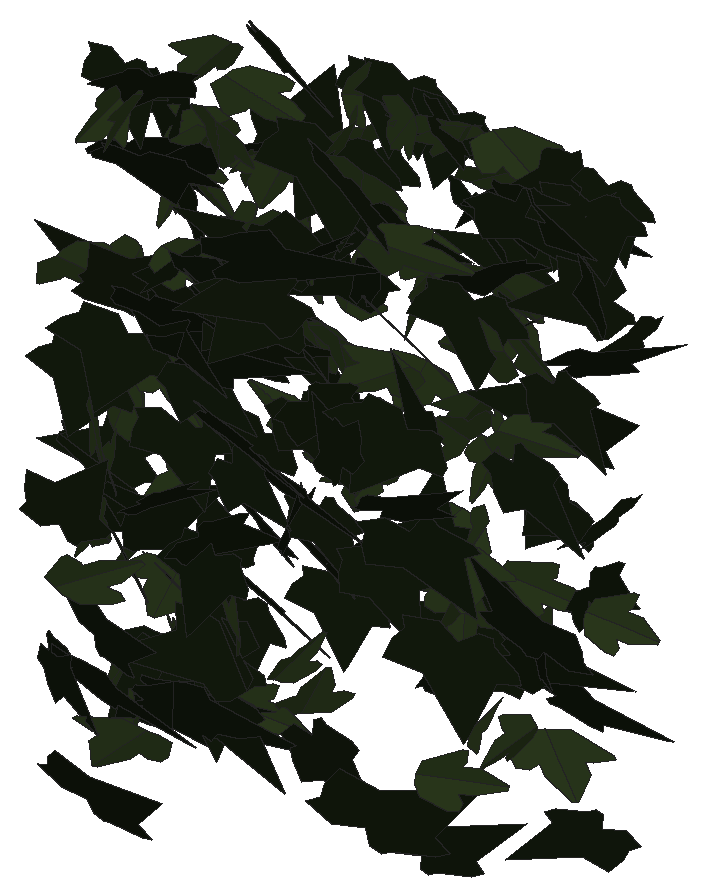
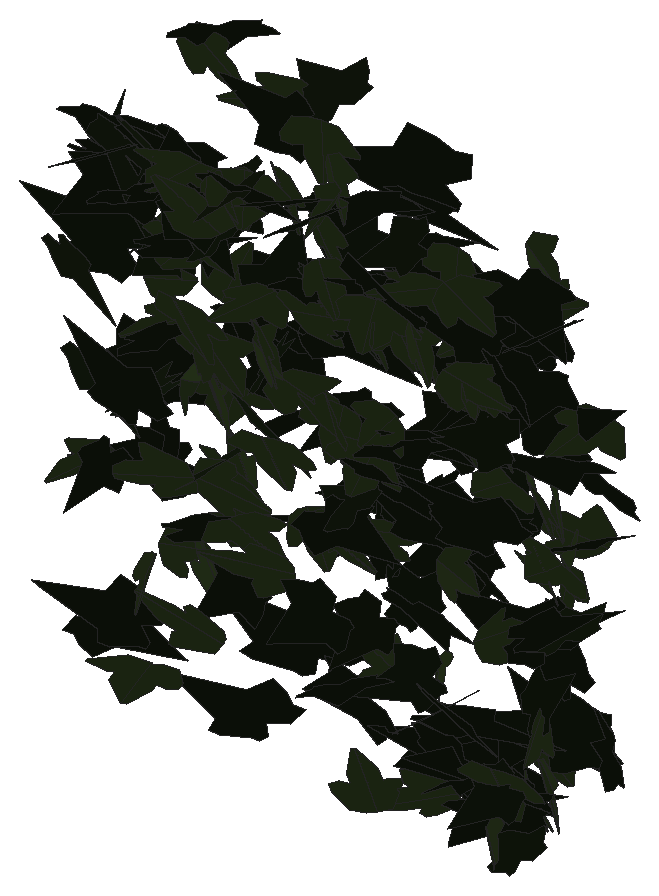
# SketchUp Ruby script. Lengths in millimetres.
U = 1.mm
M = Sketchup.active_model
def pt(a) = Geom::Point3d.new(a.map { |v| v * U })
def face(e, loops, mat)
  f = e.add_face(loops[0].map { |a| pt(a) })
  loops[1..].each { |l| e.add_face(l.map { |a| pt(a) }).erase! }
  f.material = f.back_material = mat if mat
  f
end
# faces: each face lists its corners as indices into pts; further lists are holes
def faces(e, pts, list, mat = nil) = list.each { |f| face(e, (f[0].is_a?(Array) ? f : [f]).map { |l| l.map { |i| pts[i] } }, mat) }
# xy, xz, yz: faces in a plane at the given z, y or x. An outline is a flat list of corners, or four numbers for a rectangle; further outlines are holes
def ring(l) = l.size == 4 ? [[l[0], l[1]], [l[2], l[1]], [l[2], l[3]], [l[0], l[3]]] : l.each_slice(2).to_a
def flat(e, list, mat, &to3) = list.each { |f| face(e, (f[0].is_a?(Array) ? f : [f]).map { |l| ring(l).map { |u, v| to3.(u, v) } }, mat) }
def xy(e, z, list, mat = nil) = flat(e, list, mat) { |x, y| [x, y, z] }
def xz(e, y, list, mat = nil) = flat(e, list, mat) { |x, z| [x, y, z] }
def yz(e, x, list, mat = nil) = flat(e, list, mat) { |y, z| [x, y, z] }
def lines(e, pts, list) = list.each { |a, b| e.add_line(pt(pts[a]), pt(pts[b])) }
# prism: a flat outline (further loops are holes) pulled along v
def prism(e, loops, v, mat = nil)
  f = face(e, loops, mat); d = Geom::Vector3d.new(v.map { |x| x * U })
  f.pushpull(f.normal.samedirection?(d) ? d.length : -d.length)
end
def box(e, o, s, mat = nil) = prism(e, [[o, [o[0] + s[0], o[1], o[2]], [o[0] + s[0], o[1] + s[1], o[2]], [o[0], o[1] + s[1], o[2]]]], [0, 0, s[2]], mat)
def at(x, y, z, deg = 0) = Geom::Transformation.translation(pt([x, y, z])) * Geom::Transformation.rotation(ORIGIN, Z_AXIS, deg.degrees)
def axes(o, x, y, z) = Geom::Transformation.new([*x, 0, *y, 0, *z, 0, *pt(o).to_a, 1])
def part(name) = M.definitions.add(name)
# library, detail: a bought-in or finely detailed component or shape, given as its bounding box
def library(name, o, s) = part(name).tap { |d| box(d.entities, o, s) }
def detail(e, o, s) = box(e.add_group.entities, o, s)
def put(e, d, t, mat = nil) = e.add_instance(d, t).tap { |i| i.material = mat if mat }
def group(e, t, mat = nil) = e.add_group.tap { |g| g.transformation = t; g.material = mat if mat }.entities
root = M.entities
M.materials.add("efeu1").color = [18, 25, 13]
M.materials.add("efeu2").color = [43, 57, 29]
c1 = part("ivyleaf_9")
p = [[39.1,54.8,31.7],[34.5,51.8,30.2],[-5.3,25.2,17.3],[-17.9,28.3,20.9],[-21.6,21.7,17],[-20.2,4.3,5.3],
  [-22.9,-0.3,2.5],[-17.1,-4,-0.6],[-2,-2.1,-1.2],[-0.7,-15.4,-10.1],[16.6,-22.3,-16.7],[21.1,-15.1,-12.5],
  [32.7,-10.7,-11],[46.1,-1.8,-6.6],[30.8,11.2,3.8]]
faces(c1.entities,p,[[0,1,2,3,4,5,6,7,8,9,10,11,12,13,14]],"efeu1")
c2 = part("ivyleaf_10")
p = [[0,12.8,-0.8],[-1.5,51.3,-10.9],[-4.9,51,-11.6],[-13.6,26.5,-7.3],[-13.2,15.9,-4.6],[-21.1,19.3,-7.2],
  [-29.5,16.3,-8.3],[-29.2,8.3,-6.2],[-19.7,-9.8,0.5],[-7.6,-13,4],[1,-12.2,5.8],[-0.4,51.1,-11.1],
  [-1.5,51.1,-10.9],[1,-12.4,5.9],[16.9,-12.4,3.5],[35.1,9.1,-5.1],[35,12.9,-6.1],[20.5,16.4,-4.9],
  [15.8,15,-3.8],[15.3,27.6,-7.1],[12.8,31.3,-7.8]]
faces(c2.entities,p,[[0,1,2,3,4,5,6,7,8,9,10],[11,12,0,13,14,15,16,17,18,19,20]],"efeu2")
put(root,c1,axes([5512.2,727.9,3383.8],[-0.13252,-1.17881,0.07972],[-0.00116,-0.07982,-1.18086],[2.24864,-0.06951,0.00409]))
put(root,c2,axes([5531.2,716.1,3146.5],[1.27078,-0.95438,0.07013],[0.07944,-0.05639,-1.16476],[1.81955,0.66901,0.00188]))
put(root,c1,axes([5537.2,633.9,3034.5],[-1.01754,-1.05883,0.3155],[-0.00054,-0.35036,-1.17632],[2.10271,-0.51247,0.15237]))
put(root,c1,axes([5526.2,783.4,3340.5],[-0.99944,0.03385,-1.03029],[1.91291,-0.23997,-0.52018],[-0.4357,-1.13123,0.07952]))
put(root,c1,axes([5572,679.8,2911.2],[-0.74,-0.15956,1.27167],[-1.90352,-0.7932,-0.40533],[1.52527,-1.06732,0.11112]))
put(root,c1,axes([5542.4,700.6,3305.1],[1.32687,0.89042,-0.05971],[-0.03543,-0.06124,-1.13065],[-1.69808,0.69704,-0.02307]))
put(root,c2,axes([5531.4,597.9,3193.9],[-1.11357,-0.5992,-0.91061],[1.1456,0.68404,-0.83688],[1.72964,-0.83884,-0.03197]))
put(root,c2,axes([5553.4,657.8,3375.6],[0.26095,0.41133,-1.16672],[-0.63142,-1.11863,-0.43336],[-2.2682,0.35873,-0.01359]))
put(root,c2,axes([5554.2,678.3,2790.1],[-0.03114,-0.60966,-1.0137],[0.17755,1.00997,-0.60892],[2.24429,-0.08836,0.03411]))
put(root,c2,axes([5529.6,675.3,3023.9],[1.76327,-0.17198,0.81089],[1.5071,-0.1759,-0.94206],[0.4664,1.21859,-0.02154]))
put(root,c1,axes([5538.6,648.5,2908.2],[-0.17529,-1.05107,0.83425],[0.48012,-0.83486,-1.02399],[2.50838,0.08635,0.2543]))
put(root,c1,axes([5582.3,685,3412.5],[0.33493,0.97332,-0.77439],[-0.2593,-0.76231,-0.9891],[-2.35296,0.22255,-0.00123]))
put(root,c2,axes([5571.2,748.2,3240.6],[1.16552,-0.96879,0.09099],[0.07584,-0.08245,-1.14607],[1.85036,0.61361,-0.01034]))
put(root,c1,axes([5535.4,780.1,3243.5],[1.4862,-0.6817,0.42925],[0.59094,-0.29694,-1.03643],[1.41474,0.84017,-0.01802]))
put(root,c2,axes([5578,734,2732.6],[2.16816,-0.12358,-0.14672],[-0.27506,0.02812,-1.14583],[0.24007,1.14828,0.01227]))
put(root,c1,axes([5596.4,641.2,2778.9],[0.18517,-0.91045,0.92088],[-0.09628,0.9201,0.91503],[-2.4627,-0.10443,0.03347]))
put(root,c2,axes([5599.5,785,3314.6],[-0.70687,-0.62185,0.894],[-0.69244,-0.81944,-0.72113],[1.9535,-0.51547,0.06788]))
put(root,c2,axes([5570.4,649.4,2973.9],[1.62253,-0.79065,0.01438],[-0.0173,0.01134,1.16272],[-1.50491,-0.85257,0.00213]))
put(root,c1,axes([5618.6,627.4,3164.2],[0.43411,-0.02764,1.34009],[-2.50693,0.24697,0.2293],[-0.47214,-1.33674,0.01465]))
put(root,c2,axes([5595.1,724.3,2642.3],[0.17713,-0.01007,-1.11887],[-0.50576,1.09041,-0.03192],[2.06859,0.26746,0.088]))
put(root,c1,axes([5560.1,739.4,2726.4],[1.93704,-0.46994,-0.30845],[-0.53555,0.12637,-1.12103],[0.92614,1.05596,-0.00311]))
put(root,c2,axes([5558.1,611.9,2984.7],[0.23797,-0.45101,1.17667],[1.55541,-0.87103,-0.4207],[1.82554,0.80093,0.20506]))
put(root,c1,axes([5550.1,546.1,2698.4],[0.16552,-0.22108,-1.27596],[2.39043,-0.29695,0.13706],[-0.60004,-1.24397,0.19405]))
put(root,c2,axes([5596.6,615.6,2678],[0.71983,-1.08268,-0.50877],[-0.2415,0.49427,-1.14616],[2.26389,0.39698,0.0395]))
put(root,c2,axes([5592.5,764.3,3299.9],[-0.00034,-0.92288,0.72446],[0.31149,-0.71739,-0.91384],[2.21112,0.10092,0.12885]))
put(root,c1,axes([5568.4,701.6,2609],[0.13885,-0.79141,0.86504],[0.44291,-0.8397,-0.78785],[2.187,0.2203,0.10463]))
put(root,c2,axes([5614.9,770.9,3424.3],[-0.64439,-0.9713,0.66241],[-0.31568,-0.64297,-1.02758],[2.21515,-0.37418,0.04625]))
put(root,c2,axes([5607.7,619.5,3416.9],[0.47655,-1.1291,0.45866],[0.12416,-0.45515,-1.15608],[2.31611,0.25672,-0.0324]))
put(root,c1,axes([5612.7,604.5,3116.7],[-1.6485,-0.93476,-0.12222],[0.14637,0.09536,-1.27435],[1.7882,-0.86954,-0.00837]))
put(root,c1,axes([5606.6,641.3,3334.6],[2.03483,0.62461,-0.33341],[-0.55804,-0.15903,-1.2382],[-1.22654,1.10859,0.01023]))
put(root,c1,axes([5626.7,663.8,2655.6],[-1.50662,-0.77595,0.34486],[-0.40049,-0.2775,-1.10743],[1.56565,-0.81767,0.04858]))
put(root,c1,axes([5599.4,700.7,2667.5],[-0.49343,-0.77181,-0.90761],[0.54083,0.86198,-0.81419],[2.20204,-0.38465,-0.00341]))
put(root,c2,axes([5598,742.9,3278.5],[-1.21878,0.50121,-0.81827],[1.22046,-0.5083,-0.8132],[-1.35857,-0.90626,0.00355]))
put(root,c2,axes([5625.8,528.3,2908.6],[0.01641,-0.92068,-0.76166],[0.31065,0.75545,-0.91133],[2.25282,-0.09746,0.13121]))
put(root,c2,axes([5627.5,691.2,2892.7],[-0.06818,-0.00062,1.24994],[0.32816,-1.2385,0.00433],[2.35614,0.17248,0.03557]))
put(root,c1,axes([5586.8,739.3,3076.1],[0.05617,-0.18475,1.15442],[2.12536,-0.33733,-0.08253],[0.65856,1.10443,0.16791]))
put(root,c2,axes([5632.5,763.8,3025.4],[0.15091,-0.88728,0.75288],[0.14028,-0.74928,-0.8908],[2.21022,0.10814,0.00513]))
put(root,c2,axes([5626.7,602.3,2634.8],[1.2012,-0.95708,0.418],[0.43526,-0.34989,-1.14645],[1.93942,0.67131,-0.0016]))
put(root,c1,axes([5666.8,724.1,2789.6],[-1.86407,0.45716,-0.48242],[-0.83353,0.20228,1.08088],[0.95143,1.0729,0.00177]))
put(root,c2,axes([5665.3,512.6,3001.1],[-0.16724,0.27007,1.15744],[-1.47218,0.86816,-0.2613],[-1.71738,-0.77051,0.11128]))
put(root,c1,axes([5608.3,611.3,2858.2],[-0.30899,-0.17523,1.44747],[2.65335,0.40773,0.20573],[-0.81241,1.39831,0.1214]))
put(root,c1,axes([5594.2,540.3,2694.2],[1.72987,-0.64915,0.79734],[1.26551,-0.44059,-1.1167],[1.49252,1.12596,0.02272]))
put(root,c1,axes([5677.1,652.3,3284],[0.09643,0.17666,-1.12335],[-2.01283,0.42052,0.01843],[0.79527,1.0429,0.18286]))
put(root,c1,axes([5624.6,680.8,3317.1],[0.71136,1.11165,-0.63344],[0.20247,0.63063,1.16949],[2.42663,-0.37849,0.08812]))
put(root,c1,axes([5631.7,527.7,2761.7],[0.10852,-0.08152,1.19859],[0.98302,-1.08171,-0.09814],[2.06431,0.51939,-0.01627]))
put(root,c2,axes([5696.9,517,2655.8],[-1.6113,-0.61483,0.59175],[-0.84877,-0.39188,-1.04522],[1.38462,-0.9557,0.0479]))
put(root,c1,axes([5693.7,767.1,3193.7],[-1.84149,-0.49524,0.21957],[-0.32049,-0.15222,-1.08542],[0.97994,-0.98043,0.05762]))
put(root,c1,axes([5664.9,419.8,2972.5],[-1.355,0.76537,0.62727],[0.78721,-0.47184,1.04519],[1.71096,0.82324,0.01588]))
put(root,c2,axes([5650.2,626.2,3079.4],[1.66386,-0.10146,0.7759],[1.46377,-0.10293,-0.88005],[0.27439,1.16435,-0.01019]))
put(root,c1,axes([5692.5,755.5,2946.4],[-1.95761,-0.11762,-0.46549],[0.88586,0.02562,-1.03499],[0.2241,-1.12872,0.02502]))
put(root,c2,axes([5693.3,750.7,3330.9],[0.07907,-1.21034,-0.09889],[0.02269,0.09935,-1.21096],[2.31109,0.04043,0.01527]))
put(root,c1,axes([5673,627.3,3008.8],[-0.38087,-1.12042,-0.36539],[0.12671,0.35928,-1.13815],[2.23933,-0.21089,0.00225]))
put(root,c2,axes([5704.3,664.6,3395.4],[-1.85276,0.59265,0.33026],[-0.58105,0.13317,-1.13889],[-1.15312,-1.01933,0.04323]))
put(root,c1,axes([5658.3,590.1,2657.7],[0.51358,0.68474,-1.10394],[0.62141,1.05556,0.73454],[2.393,-0.42106,0.04618]))
put(root,c1,axes([5685.9,665.3,2661.4],[-0.47163,-1.17538,-0.04486],[0.01717,0.04394,-1.20122],[2.23854,-0.24797,-0.00024]))
put(root,c1,axes([5744.8,640.6,2721.1],[-1.96274,-0.12095,0.87929],[-1.64089,-0.18364,-1.03647],[0.40121,-1.34275,0.06254]))
put(root,c1,axes([5700.2,788,3184.8],[-1.22595,-0.99297,0.05727],[-0.05926,-0.04806,-1.18361],[1.89204,-0.6449,0.00004]))
put(root,c2,axes([5668.5,751.7,3404.2],[-1.098,-0.39967,-0.9265],[1.86491,0.03275,-0.62429],[0.45824,-1.09095,0.32069]))
put(root,c2,axes([5685.1,419.3,2895.9],[-0.68509,-0.62765,0.98561],[0.84543,0.88038,0.72287],[-2.0569,0.5709,-0.03116]))
put(root,c1,axes([5731,554.1,3272.8],[-0.65864,1.1536,0.10618],[-0.08204,0.09791,-1.20432],[-2.20329,-0.3485,0.01311]))
put(root,c1,axes([5660.1,731.4,3059.3],[0.21845,-0.1723,1.27264],[2.36092,-0.31577,-0.15463],[0.6325,1.23817,0.13766]))
put(root,c1,axes([5686.5,763.2,3468.1],[1.65908,-0.77447,-0.11836],[-0.15619,0.08583,-1.16603],[1.48287,0.87554,0.00961]))
put(root,c2,axes([5730.8,741.9,3325.1],[-1.16727,-0.93341,0.32222],[-0.06044,-0.36047,-1.10466],[1.87836,-0.59165,0.16469]))
put(root,c1,axes([5685.6,445.6,2600.4],[-0.43614,-0.31013,1.32319],[1.7511,-1.023,-0.08042],[1.90365,0.86996,0.37713]))
put(root,c2,axes([5704.5,586.3,3262],[0.95155,0.59753,0.91656],[0.76319,0.83753,-0.76475],[-1.93746,0.62338,0.14891]))
put(root,c1,axes([5714.1,694.2,2758.4],[-0.26294,-1.28206,0.33169],[-0.09692,-0.3281,-1.2894],[2.51849,-0.14648,-0.01499]))
put(root,c2,axes([5720.9,696.6,3273],[1.11341,-0.92526,0.45871],[0.55609,-0.35736,-1.09347],[1.88517,0.65189,0.05163]))
put(root,c1,axes([5672.4,602,2659.4],[1.18844,0.40686,-1.26793],[2.02021,0.69347,0.74529],[1.5302,-1.23153,0.00079]))
put(root,c1,axes([5718,522.7,3233.3],[2.41785,0.34341,-0.24807],[-0.45706,-0.06221,-1.31601],[-0.66419,1.29291,0.00257]))
put(root,c1,axes([5696,551.3,3204.1],[-0.04366,0.0327,-1.28813],[2.44784,0.07876,-0.02091],[0.14881,-1.28593,-0.03403]))
put(root,c1,axes([5722.8,500.9,2981],[1.11202,0.60526,0.85788],[0.89138,0.72841,-0.83292],[-1.78834,0.73943,0.11829]))
put(root,c2,axes([5730.5,766.9,3201.5],[-1.63095,0.60816,-0.35576],[0.49955,-0.2443,-1.04987],[-1.24442,-0.89513,0.04482]))
put(root,c2,axes([5719.6,675.8,2633.4],[0.45657,0.45907,1.08431],[1.0859,0.92267,-0.51687],[-1.96032,0.61803,-0.03377]))
put(root,c2,axes([5761.6,618.9,2772.3],[0.21466,0.0952,-1.13734],[-0.39559,1.12548,0.07359],[2.13582,0.19889,0.12794]))
put(root,c1,axes([5728.4,758.4,3111.4],[-0.891,-0.47412,-0.89524],[1.67817,0.29482,-0.61725],[0.94921,-0.96629,0.25093]))
put(root,c2,axes([5756.9,760.2,3346.7],[-2.00461,-0.36926,-0.11006],[0.21274,0.01375,-1.11588],[0.7018,-1.05893,0.02389]))
put(root,c1,axes([5758.8,747.8,3357.3],[-1.98321,0.79256,0.39181],[0.59389,-0.23695,1.3092],[1.57437,1.08776,-0.0003]))
put(root,c1,axes([5721.9,626.9,2661.5],[-0.55267,-0.12194,-1.27016],[2.32873,0.34291,-0.31266],[0.68888,-1.257,0.03792]))
put(root,c2,axes([5792.1,723.6,3003],[1.19994,0.18419,0.91532],[-1.72717,-0.13873,0.65302],[0.4177,-1.10276,0.07073]))
put(root,c1,axes([5745.3,552.6,3144.1],[0.8078,-0.76433,-1.01895],[-0.6468,0.96715,-0.86703],[2.33634,0.53202,0.11227]))
put(root,c1,axes([5730.1,681.6,2800.6],[1.96318,-0.60704,0.03],[0.04357,-0.02025,-1.19687],[1.15591,1.03175,-0.00584]))
put(root,c1,axes([5762.2,558.2,2923.9],[-0.159,0.41063,-1.21943],[-0.32794,1.20742,0.4184],[2.42681,0.19007,-0.02335]))
put(root,c2,axes([5775.6,667.4,3296.2],[0.19629,-0.98126,0.73885],[0.19604,-0.73193,-0.98644],[2.3295,0.14428,0.02076]))
put(root,c1,axes([5777.2,560.5,2899.1],[-1.97885,0.04671,-0.76432],[1.44612,-0.09692,-1.03957],[-0.18074,-1.28681,0.05056]))
put(root,c2,axes([5776.9,745.3,3124.6],[-2.04092,0.30855,-0.10582],[0.18956,-0.03652,-1.11584],[-0.59116,-1.07695,0.00752]))
put(root,c1,axes([5748.4,678.6,2886.2],[0.09528,-0.49492,1.10131],[0.70239,-1.04323,-0.4856],[2.18796,0.35646,0.10793]))
put(root,c2,axes([5782.4,732.4,2631.6],[-0.8488,-1.08893,0.01604],[0.04012,0.0087,1.17661],[-2.07229,0.44619,0.01621]))
put(root,c1,axes([5839.6,632.8,3279.5],[-0.71733,0.14768,1.21148],[-2.25425,0.26138,-0.40037],[-0.55992,-1.24154,0.05982]))
put(root,c1,axes([5743.1,548.6,3157.3],[0.9154,-0.06964,1.19668],[2.27995,-0.01764,-0.48252],[0.08062,1.2896,0.05802]))
put(root,c1,axes([5797.9,585.4,3241.6],[-0.85733,-0.94656,0.77094],[-0.40002,-0.74934,-1.04286],[2.28871,-0.48554,0.10651]))
put(root,c1,axes([5760,561.9,3086.2],[2.37821,-0.56664,0.11152],[0.19723,-0.0415,-1.37205],[1.08128,1.25386,0.00499]))
put(root,c1,axes([5773.2,772.1,3063.3],[0.51907,-1.00568,0.65559],[0.29276,-0.63748,-1.04189],[2.26594,0.31274,-0.01557]))
put(root,c1,axes([5790,584.2,3015.5],[0.70696,-0.75058,-0.78672],[-0.5295,0.73808,-0.83553],[2.00053,0.4606,0.05687]))
put(root,c1,axes([5824,764.7,3034],[-0.23205,0.41848,-1.08834],[-0.00849,-1.09444,-0.42032],[-2.21916,-0.03957,0.11542]))
put(root,c1,axes([5794.9,703.6,2870.1],[1.95661,-0.31088,-0.48295],[-0.86166,0.1707,-1.07363],[0.67265,1.12295,0.0295]))
put(root,c2,axes([5791.9,711,3277.5],[0.95421,-0.6935,0.82637],[1.18954,-0.556,-0.84582],[1.67349,0.79064,0.13003]))
put(root,c1,axes([5816.6,736.2,3361.5],[-1.3674,-0.88693,0.24554],[-0.02054,-0.30337,-1.12739],[1.75139,-0.69603,0.17849]))
put(root,c2,axes([5822.1,774.9,3385.2],[-0.65554,-1.06513,0.02709],[-0.03556,-0.02243,-1.11938],[2.02749,-0.34478,-0.01087]))
put(root,c2,axes([5813.6,770.3,3163.4],[1.74872,-0.66379,0.16953],[-0.25742,0.10228,1.13351],[-1.27821,-0.92873,0.00366]))
put(root,c1,axes([5769.9,550.3,3267.1],[0.94407,-0.24499,1.08564],[1.78621,-0.54673,-0.5522],[1.1384,1.06101,-0.03387]))
put(root,c1,axes([5818,748.1,2786.6],[-0.68048,-1.12686,-0.05529],[0.03962,0.0514,-1.18222],[2.14685,-0.35813,0.00429]))
put(root,c1,axes([5828,642.6,2916.2],[0.2422,0.84899,0.91133],[-0.85012,-0.82403,0.83003],[2.21278,-0.40951,0.21914]))
put(root,c2,axes([5870.5,716.7,2980.2],[0.79673,-0.24248,-1.02857],[-1.63327,0.56761,-0.48308],[1.17367,0.95448,0.02598]))
put(root,c1,axes([5820.2,669.1,3062.5],[0.50969,-1.07085,-0.629],[-0.27769,0.61187,-1.10381],[2.34724,0.30492,0.006]))
put(root,c1,axes([5870.2,693.3,3258.7],[0.23346,0.244,-1.19804],[-1.07593,-1.0563,-0.27301],[-2.06324,0.57844,0.00681]))
put(root,c2,axes([5846.7,732.1,3461.4],[-0.17838,0.50593,1.05973],[-0.56967,1.01769,-0.51233],[-2.16111,-0.31002,0.04758]))
put(root,c1,axes([5837.2,773.4,3363.9],[-1.06888,-0.93242,-0.28042],[0.29354,0.23445,-1.08844],[1.8297,-0.58232,0.0108]))
put(root,c2,axes([5851.9,710.3,3140.2],[-2.04992,0.43506,0.1365],[-0.24049,0.05162,-1.16164],[-0.83381,-1.08448,-0.00054]))
put(root,c2,axes([5879.5,742.1,3290.5],[1.16722,0.12514,1.01312],[-1.93559,-0.02699,0.61899],[0.16749,-1.18398,0.09297]))
put(root,c2,axes([5839.4,619.3,2746.1],[-0.02358,-1.00098,0.5724],[0.1022,0.57131,1.00024],[-2.19217,0.0374,0.04048]))
put(root,c1,axes([5820,733.4,3299.2],[0.06737,-0.69826,0.98523],[1.00618,-0.87721,-0.64069],[2.0663,0.44992,0.27986]))
put(root,c1,axes([5814.1,617.4,3000.3],[1.88575,-0.55712,0.409],[0.67583,-0.20295,-1.13671],[1.12846,1.05254,-0.0027]))
put(root,c1,axes([5888.1,700.8,3314.1],[-1.25448,1.03517,0.04247],[-0.04653,0.03478,-1.22721],[-1.97125,-0.65959,0.00194]))
put(root,c1,axes([5846.5,787.3,3453.7],[-0.33188,-1.12238,0.16708],[-0.00686,-0.16849,-1.13564],[2.15965,-0.17302,0.02207]))
put(root,c1,axes([5856.3,720.9,2864.8],[0.98581,0.7125,0.80387],[0.92482,0.64049,-0.8808],[-1.82325,0.71012,-0.01213]))
put(root,c1,axes([5853.8,661.2,2945.2],[0.30352,-1.14754,-0.25465],[-0.09636,0.25004,-1.15847],[2.23505,0.16662,-0.01536]))
put(root,c2,axes([5889.7,694.6,3390.1],[1.1713,-0.66524,-0.76576],[-0.70299,0.68721,-0.89387],[1.79799,0.70206,0.14936]))
put(root,c2,axes([5885.6,717.6,2983.2],[-0.95789,-1.08122,0.11806],[-0.0895,-0.10834,-1.19262],[2.06807,-0.50549,0.00307]))
put(root,c1,axes([5868.6,668.8,3426.7],[-1.20229,-1.30854,-0.39119],[0.2985,0.35865,-1.45298],[2.58212,-0.65074,-0.01418]))
put(root,c1,axes([5893.4,516.3,3291.7],[-1.67202,-0.8025,0.25143],[-0.33701,-0.17892,-1.18982],[1.56463,-0.89611,0.0124]))
put(root,c2,axes([5888.3,670.7,3461.7],[0.23966,-1.20228,-0.28586],[-0.0179,0.2864,-1.20869],[2.35189,0.12469,0.01993]))
put(root,c1,axes([5870.9,624.4,3110.9],[0.09322,-0.17499,-1.20851],[-0.33132,1.19612,-0.18025],[2.30027,0.17938,0.02301]))
put(root,c1,axes([5929.5,496.7,3330.3],[-2.18823,-0.04668,0.44239],[-0.84205,-0.00738,-1.15067],[0.08796,-1.23191,-0.00987]))
put(root,c1,axes([5884.4,784.9,3467.9],[-0.70812,-1.06839,-0.03902],[0.46551,-0.04485,-1.10434],[1.98075,-0.37141,0.24559]))
put(root,c1,axes([5897.5,580.2,3332.6],[0.79126,0.77698,0.75727],[0.62197,0.68362,-0.88084],[-1.96902,0.52818,0.02608]))
put(root,c2,axes([5937.8,694.1,3146.8],[-1.14018,-0.43431,0.86331],[-1.02736,-0.69212,-0.72278],[1.52558,-0.79068,0.15848]))
put(root,c2,axes([5913.1,770.8,3103.8],[2.09562,0.01348,-0.19923],[-0.37997,0.09441,-1.09705],[0.00684,1.11499,0.0953]))
put(root,c1,axes([5914.3,670.9,3256.2],[-0.13887,-0.38498,1.2195],[1.15432,1.06495,0.37248],[-2.14271,0.59866,0.12162]))
put(root,c2,axes([5926.3,727.5,3459.9],[1.27635,-0.87257,-0.43411],[-0.30203,0.42215,-1.0937],[1.83008,0.67822,0.12226]))
put(root,c1,axes([5876,477.6,3363.7],[1.19486,0.10855,1.36523],[2.5522,0.25627,-0.63705],[-0.52933,1.48065,0.01017]))
put(root,c1,axes([5891.8,605.6,2680.2],[-0.26996,-0.21312,-1.29929],[2.49343,0.10716,-0.16061],[0.24928,-1.30261,0.19936]))
put(root,c2,axes([5942.5,751.8,3244.7],[0.86669,-0.97498,-0.46531],[-0.31947,0.43497,-1.07568],[2.0311,0.48445,0.02936]))
put(root,c2,axes([5934,756.8,3228.9],[0.55543,-0.99703,0.70379],[0.47087,-0.66028,-1.03797],[2.27445,0.38018,0.04302]))
put(root,c2,axes([5971.4,598.6,3454.1],[-2.10685,0.21609,0.30852],[-0.56579,0.0869,-1.12757],[-0.44021,-1.1459,-0.02733]))
put(root,c2,axes([5967.8,753.2,3452.2],[-1.89978,-0.5519,-0.00445],[0.00346,0.00591,-1.14061],[1.05041,-0.99819,-0.00429]))
put(root,c1,axes([5960.8,772.7,3455.9],[-1.77219,-0.40484,-0.51126],[0.98554,0.08271,-1.00864],[0.75442,-1.05906,0.11666]))
put(root,c2,axes([5948,738.5,3287.7],[-0.90257,-0.59648,-0.83533],[1.41739,0.43327,-0.73219],[1.34432,-0.85729,0.21116]))
put(root,c2,axes([5983.8,757.3,3449.1],[-0.93523,-1.01638,0.13027],[-0.1414,-0.10876,-1.12877],[1.94506,-0.4966,-0.01942]))
put(root,c1,axes([5959.2,747.4,3463.9],[1.50348,-0.46809,-0.71031],[-0.83658,0.60529,-0.88775],[1.3861,0.87305,0.23465]))
put(root,c2,axes([5988,736,2949.7],[1.50522,0.57138,-0.69021],[-1.07146,-0.39933,-0.97568],[-1.32667,0.97078,0.00489]))
put(root,c2,axes([5947.5,716.4,2891.2],[-0.19557,-0.02246,-1.13855],[2.1607,0.08714,-0.10418],[0.16903,-1.13985,0.01447]))
put(root,c1,axes([6000.9,640.4,3232],[1.78699,-0.92333,-0.10896],[0.14981,-0.07536,1.31687],[-1.76313,-0.94223,0.00146]))
put(root,c1,axes([5977.9,553.1,3475.6],[0.28822,-1.07001,0.92119],[0.62402,-0.87449,-1.06967],[2.61369,0.32678,0.1538]))
put(root,c1,axes([6030.5,638.1,3107.7],[-0.47084,-0.90175,0.94208],[0.40513,0.9181,0.9347],[-2.44867,0.32529,-0.0265]))
put(root,c1,axes([6041.8,465.9,3160.2],[-0.05441,0.3249,1.19048],[-0.43509,1.16879,-0.32447],[-2.30793,-0.228,0.03311]))
put(root,c1,axes([5998.5,763.7,3364],[0.52969,-1.01535,0.42906],[0.19406,-0.41692,-1.05275],[2.08888,0.2962,-0.011]))
put(root,c1,axes([6044.6,761.1,3392.6],[-0.24126,0.98364,-0.56421],[0.08667,-0.56285,-0.9915],[-2.15643,-0.13267,0.02327]))
put(root,c2,axes([6012,772.1,3389.5],[-0.92049,-0.87192,0.56299],[1.04887,0.31056,0.95444],[-1.67381,0.67411,0.28848]))
put(root,c1,axes([6045.2,651.8,2815.2],[-0.27853,0.40003,-1.17061],[-0.85604,1.08089,0.4256],[2.19327,0.47268,0.01746]))
put(root,c1,axes([6067.2,584.6,2997.2],[-1.97503,0.99524,-0.4144],[-0.58316,0.27919,1.43782],[1.96716,1.08199,0.01017]))
put(root,c2,axes([6062.4,692.1,3152.2],[-0.53432,-1.09173,0.38776],[-0.22203,-0.37031,-1.12708],[2.19375,-0.30339,-0.01963]))
put(root,c2,axes([6067.9,746.5,3231.4],[2.06209,-0.49228,-0.32428],[-0.50817,0.1951,-1.18831],[1.00022,1.11402,0.06482]))
put(root,c1,axes([6035,558.3,3055.6],[1.73036,0.73917,0.00032],[-0.00753,0.00435,1.17173],[1.40676,-0.90917,0.00587]))
put(root,c1,axes([6047.6,531.5,2999.9],[0.02385,-1.20688,-0.41496],[0.01797,0.41505,-1.20688],[2.42885,0.00878,0.013]))
put(root,c2,axes([6108.1,639.7,2926.4],[-0.17919,0.06695,-1.24568],[-1.94022,0.71586,0.11552],[1.36836,1.02379,0.00068]))
put(root,c2,axes([6044.5,763.7,3452.3],[1.4516,0.62275,0.63122],[0.91544,0.40889,-0.9846],[-1.41772,0.90166,0.01053]))
put(root,c1,axes([6026,566.9,3424],[1.57806,-0.06966,-0.82887],[1.57371,0.19614,0.81068],[0.17193,-1.15589,0.18751]))
put(root,c2,axes([6030,752.9,2787.6],[0.75327,-0.11197,-1.11121],[2.05157,-0.27005,0.41116],[-0.55594,-1.14826,0.01166]))
put(root,c1,axes([6108.7,751.8,3312],[-0.88637,-0.90928,-0.57736],[-0.47682,-0.52031,1.02154],[-1.9937,0.52869,0.01237]))
put(root,c1,axes([6089.5,521.2,3196.2],[-2.07464,-0.59876,-0.10389],[0.19204,0.03205,-1.24353],[1.14052,-1.09455,0.02041]))
put(root,c1,axes([6038.7,522.6,2654],[-0.65133,-0.01738,1.47751],[2.80478,-0.114,0.34001],[0.20393,1.51233,0.04261]))
put(root,c2,axes([6095.8,702.5,3102.9],[-0.11488,0.67451,-0.93926],[-0.54334,0.90273,0.66663],[2.13266,0.26632,0.11924]))
put(root,c1,axes([6094.9,655.1,3349.5],[0.91982,1.3041,-0.01607],[-0.03427,-0.01047,-1.39071],[-2.48192,0.48345,0.01325]))
put(root,c1,axes([6057.4,602.2,2589.1],[-0.16058,-0.01502,1.26377],[2.35469,0.25767,0.08566],[-0.4912,1.2401,-0.00249]))
put(root,c2,axes([6080.6,709,3314],[-1.9761,-0.09092,-0.46939],[0.88244,0.08236,-1.04159],[0.22204,-1.1365,-0.03793]))
put(root,c1,axes([6132.4,656.1,2858.3],[-1.10271,-1.22091,-0.61809],[-0.53255,-0.55132,1.35133],[-2.5494,0.64326,-0.01494]))
put(root,c2,axes([6066.2,520.6,3435.3],[-0.77475,-0.14289,-1.17115],[2.10302,0.38806,-0.43143],[0.78702,-1.17759,-0.00007]))
put(root,c2,axes([6096.3,590.9,2912.8],[0.1042,-1.16952,-0.13251],[0.02756,-0.13198,1.17077],[-2.2399,-0.05603,0.00824]))
put(root,c2,axes([6097.6,615.8,2934.2],[1.97253,-0.56063,0.38974],[0.66595,-0.17223,-1.17826],[1.11588,1.09381,0.01424]))
put(root,c2,axes([6119,641.7,3120.2],[1.32919,-0.97801,0.14131],[0.15664,-0.11487,-1.20178],[1.87415,0.70323,0.00022]))
put(root,c2,axes([6152,693.1,3225.9],[-0.79871,0.52817,-0.94292],[-1.29199,0.65825,0.67085],[1.60051,0.79493,0.07099]))
put(root,c1,axes([6097.9,655.1,2956],[0.40748,-1.25302,0.05679],[0.02313,-0.05554,-1.27118],[2.38709,0.21443,0.00263]))
put(root,c2,axes([6129.9,738.9,2844.3],[-0.97318,0.92856,0.58567],[-0.56907,0.50386,-1.05991],[-2.0104,-0.59211,0.01652]))
put(root,c2,axes([6130.5,587.4,3172.8],[-0.55148,-0.7793,-0.91929],[-0.63293,-0.85707,0.83138],[-2.2046,0.441,-0.00873]))
put(root,c2,axes([6132.4,607,3045.3],[0.65105,-1.17292,-0.30443],[-0.19694,0.2869,-1.22164],[2.29784,0.35691,-0.01845]))
put(root,c1,axes([6156.1,740.5,3455.7],[-1.66886,0.74677,0.00919],[-0.057,-0.02101,-1.15122],[-1.42021,-0.87667,0.03541]))
put(root,c1,axes([6126.9,785.7,3398.3],[-0.96526,-1.03041,0.02613],[-0.09365,-0.00489,-1.1477],[1.95948,-0.50783,-0.04198]))
put(root,c1,axes([6153,729.8,3152.8],[-0.23627,-0.99125,-0.70794],[0.02144,-0.71251,0.99568],[-2.31818,0.09444,0.08136]))
put(root,c1,axes([6129.6,683.9,3272.6],[0.82594,0.61976,0.86427],[0.54219,0.83159,-0.73938],[-1.9501,0.4937,0.16048]))
put(root,c2,axes([6122.9,620.1,2772.3],[0.36625,-1.06057,-0.51515],[0.39961,-0.4828,1.0724],[-2.20813,-0.26328,0.10863]))
put(root,c1,axes([6091.2,711.9,3411.7],[1.0739,-0.2794,-1.05982],[2.08143,0.22208,0.52372],[0.13746,-1.17995,0.34953]))
put(root,c2,axes([6128,568.6,3018.7],[1.8312,0.67196,0.14092],[0.22562,0.07638,-1.17357],[-1.28707,0.96943,-0.00522]))
put(root,c1,axes([6120.1,695,3429.3],[-0.51136,-0.43023,-1.11387],[1.01844,0.97727,-0.50655],[2.03157,-0.5982,-0.02643]))
put(root,c2,axes([6130.8,742.9,2697.2],[1.72755,0.77256,0.32329],[0.46586,0.2112,-1.19196],[-1.52428,0.94013,0.00211]))
put(root,c1,axes([6124.2,494.2,3081.8],[-0.84051,-0.49958,-1.05988],[1.29677,0.81197,-0.66664],[1.8142,-0.81184,-0.01453]))
put(root,c1,axes([6114.1,785.1,3098.2],[-0.19117,0.08933,1.36953],[1.43825,-1.14268,0.12996],[2.1804,0.76157,0.03435]))
put(root,c2,axes([6143.6,655.2,3152.2],[-0.75017,-0.38346,-1.015],[1.52218,0.62706,-0.54749],[1.39542,-0.89016,0.05156]))
put(root,c1,axes([6164.5,710.7,3051.1],[-0.76697,-0.91252,0.85826],[-0.26198,-0.86386,-0.98311],[2.36973,-0.39084,0.16909]))
put(root,c1,axes([6183.3,719.5,3420.8],[0.22895,1.0288,0.50547],[0.0226,0.5071,-1.03495],[-2.18146,0.11323,0.04233]))
put(root,c1,axes([6146.7,749.2,3385.6],[1.80683,0.48409,0.42628],[0.69107,0.22583,-1.06514],[-1.01463,1.01588,0.03364]))
put(root,c2,axes([6136.9,678.7,2942.7],[0.50962,0.19879,1.12627],[1.66477,0.7096,-0.33321],[-1.40226,0.91469,0.01373]))
put(root,c1,axes([6180.5,709.2,3050.5],[-0.97648,-0.679,1.00469],[-0.37474,-1.02979,-0.79652],[2.27723,-0.46062,0.29974]))
put(root,c1,axes([6141.1,748.5,2761],[1.13707,-0.35896,0.96597],[1.66687,-0.41151,-0.69462],[1.0335,1.05863,0.05753]))
put(root,c2,axes([6193.4,610.9,2792.5],[0.07471,-0.4782,1.10118],[0.18267,-1.09699,-0.4798],[2.27753,0.10367,0.00236]))
put(root,c2,axes([6169.7,482.8,2780.1],[0.22121,0.18846,1.23176],[0.71993,1.17339,-0.21523],[-2.25965,0.39229,0.05201]))
put(root,c1,axes([6180.1,786.3,3431.3],[-0.32644,-1.13794,0.04407],[0.23186,-0.06265,-1.14346],[2.1549,-0.16564,0.12971]))
put(root,c1,axes([6202.1,479.5,2969.5],[-1.03286,-1.29529,-0.3192],[0.22415,0.29673,-1.40437],[2.52903,-0.5553,-0.00589]))
put(root,c1,axes([6204.2,720.6,3447.6],[-1.25364,-0.72747,-0.60798],[0.96611,0.35464,-0.97431],[1.52395,-0.82326,0.11753]))
put(root,c1,axes([6221.4,704.2,2953.7],[0.08526,-0.12243,-1.21855],[-1.03454,1.09068,-0.12957],[2.08864,0.54523,-0.01443]))
put(root,c1,axes([6246.3,762.4,3264],[-1.08692,1.00337,-0.11581],[0.11807,-0.09794,-1.1545],[-1.91866,-0.57443,-0.00544]))
put(root,c1,axes([6265.3,680,3358.9],[-2.02551,0.19543,0.43685],[-0.82779,0.04934,-1.0817],[-0.37993,-1.14937,0.02784]))
put(root,c1,axes([6215.6,602.5,2908.6],[-0.38151,0.15131,1.19058],[0.07873,-1.20548,0.16017],[2.28278,0.06686,0.19345]))
put(root,c1,axes([6199.5,592.7,2903.3],[0.53894,0.31598,-1.10813],[1.00753,0.97787,0.41412],[1.94792,-0.59322,0.0924]))
put(root,c2,axes([6285.1,444.1,3405],[-1.09153,0.23946,1.0873],[-2.05854,0.17013,-0.60799],[-0.50235,-1.21746,0.1289]))
put(root,c1,axes([6208.1,692.3,3250],[1.38959,1.08094,-0.29484],[0.28706,0.25389,1.30432],[2.11299,-0.74536,0.0167]))
put(root,c1,axes([6269.8,687.6,3069.8],[-1.02093,1.08861,-0.28537],[0.24462,-0.2548,-1.2136],[-2.12784,-0.55161,-0.0026]))
put(root,c1,axes([6275.6,648.9,2676.4],[-0.11594,0.11601,-1.16798],[-0.35912,-1.15531,-0.10491],[-2.20479,0.18208,0.07851]))
put(root,c1,axes([6244.4,457.1,3446.2],[-0.96217,-1.12538,-0.2733],[0.19623,0.25329,-1.23368],[2.19532,-0.51587,-0.00951]))
put(root,c1,axes([6284.1,533.1,2972.1],[1.14533,-0.63968,1.14776],[-1.48836,0.84012,0.87825],[-2.00963,-0.98677,0.00369]))
put(root,c1,axes([6257.3,670,3358.9],[-0.43268,0.02277,1.13693],[-0.53914,-1.12401,-0.03413],[2.09601,-0.28442,0.22592]))
put(root,c2,axes([6254.7,683.6,2933.1],[0.20283,0.62685,1.00119],[0.42003,0.97699,-0.63519],[-2.20855,0.24337,-0.02885]))
put(root,c1,axes([6251.7,599.5,3274.4],[0.50074,-1.12344,-0.42317],[-0.14269,0.417,-1.15365],[2.28033,0.27279,0.02073]))
put(root,c1,axes([6248.9,530.6,3200.4],[0.92211,-1.14825,-0.60892],[-0.31438,0.59018,-1.24435],[2.45357,0.50716,0.0694]))
